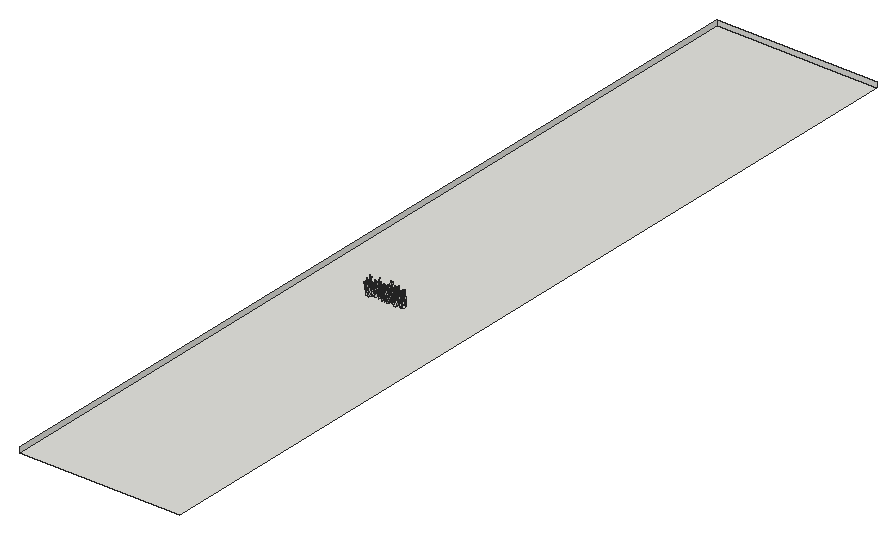
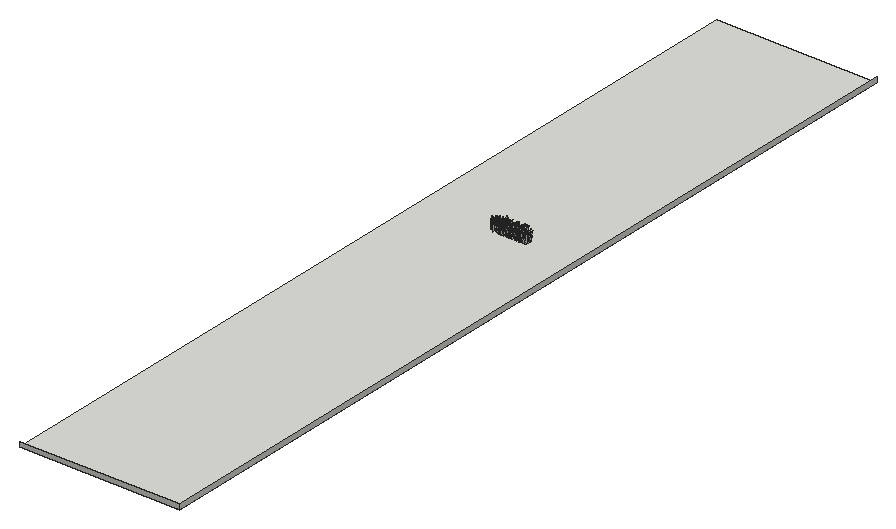
# SketchUp Ruby script. Lengths in inches.
U = 1.inch
M = Sketchup.active_model
def pt(a) = Geom::Point3d.new(a.map { |v| v * U })
def face(e, loops, mat)
  f = e.add_face(loops[0].map { |a| pt(a) })
  loops[1..].each { |l| e.add_face(l.map { |a| pt(a) }).erase! }
  f.material = f.back_material = mat if mat
  f
end
# faces: each face lists its corners as indices into pts; further lists are holes
def faces(e, pts, list, mat = nil) = list.each { |f| face(e, (f[0].is_a?(Array) ? f : [f]).map { |l| l.map { |i| pts[i] } }, mat) }
# xy, xz, yz: faces in a plane at the given z, y or x. An outline is a flat list of corners, or four numbers for a rectangle; further outlines are holes
def ring(l) = l.size == 4 ? [[l[0], l[1]], [l[2], l[1]], [l[2], l[3]], [l[0], l[3]]] : l.each_slice(2).to_a
def flat(e, list, mat, &to3) = list.each { |f| face(e, (f[0].is_a?(Array) ? f : [f]).map { |l| ring(l).map { |u, v| to3.(u, v) } }, mat) }
def xy(e, z, list, mat = nil) = flat(e, list, mat) { |x, y| [x, y, z] }
def xz(e, y, list, mat = nil) = flat(e, list, mat) { |x, z| [x, y, z] }
def yz(e, x, list, mat = nil) = flat(e, list, mat) { |y, z| [x, y, z] }
def lines(e, pts, list) = list.each { |a, b| e.add_line(pt(pts[a]), pt(pts[b])) }
# prism: a flat outline (further loops are holes) pulled along v
def prism(e, loops, v, mat = nil)
  f = face(e, loops, mat); d = Geom::Vector3d.new(v.map { |x| x * U })
  f.pushpull(f.normal.samedirection?(d) ? d.length : -d.length)
end
def box(e, o, s, mat = nil) = prism(e, [[o, [o[0] + s[0], o[1], o[2]], [o[0] + s[0], o[1] + s[1], o[2]], [o[0], o[1] + s[1], o[2]]]], [0, 0, s[2]], mat)
def at(x, y, z, deg = 0) = Geom::Transformation.translation(pt([x, y, z])) * Geom::Transformation.rotation(ORIGIN, Z_AXIS, deg.degrees)
def axes(o, x, y, z) = Geom::Transformation.new([*x, 0, *y, 0, *z, 0, *pt(o).to_a, 1])
def part(name) = M.definitions.add(name)
# library, detail: a bought-in or finely detailed component or shape, given as its bounding box
def library(name, o, s) = part(name).tap { |d| box(d.entities, o, s) }
def detail(e, o, s) = box(e.add_group.entities, o, s)
def put(e, d, t, mat = nil) = e.add_instance(d, t).tap { |i| i.material = mat if mat }
def group(e, t, mat = nil) = e.add_group.tap { |g| g.transformation = t; g.material = mat if mat }.entities
root = M.entities
c1 = part("fur_instance\#9")
p = [[0.8125,0,1.79],[0.67,-0.02,1.48],[0,-0.11,0],[0,0.11,0]]
faces(c1.entities,p,[[0,1,2,3]])
xy(root,-27.625,[[0,5.77,196.6875,1083.4]])
xz(root,1083.4,[[0,-27.625,196.6875,-21.625]])
yz(root,0,[[5.77,-27.625,1083.4,-21.625]])
put(root,c1,axes([103.26,455.89,-27.1],[-3.36255,6.42423,2.20976],[5.77924,4.00105,-2.8377],[3.57129,-0.42595,6.67271]))
put(root,c1,axes([74.56,459.28,-27.1],[-6.62778,2.24684,1.33683],[2.5489,6.36376,1.94128],[0.58185,-2.2841,6.72363]))
put(root,c1,axes([77.29,458.65,-27.1],[2.95876,-6.29379,1.88961],[-6.54545,-2.63888,1.45948],[0.58268,2.31543,6.79971]))
put(root,c1,axes([104.48,458.19,-27.1],[4.99795,-3.82327,1.26682],[-4.01963,-4.86241,1.18375],[-0.25457,1.71502,6.18026]))
put(root,c1,axes([77.6,460.84,-27.1],[6.21031,-0.46369,2.15458],[0.49806,-5.98034,-2.72263],[-2.14689,-2.7287,5.60092]))
put(root,c1,axes([84.37,459.16,-27.1],[-1.75901,-5.06572,0.78099],[-4.97011,1.48393,-1.5689],[-1.25276,1.22556,5.12778]))
put(root,c1,axes([110.68,457.23,-27.1],[-4.80095,-0.85986,1.55653],[-1.24807,4.82151,-1.18603],[1.26668,1.49164,4.73094]))
put(root,c1,axes([102.17,460.42,-27.1],[1.78326,-6.33726,0.7797],[-6.26284,-1.89367,-1.06754],[-1.24322,0.44943,6.49625]))
put(root,c1,axes([85.58,460.71,-27.1],[-2.3415,-4.6423,0.1365],[-4.37976,2.25803,1.66471],[1.54509,-0.63449,4.92568]))
put(root,c1,axes([108.52,457.49,-27.1],[-0.93822,4.8343,1.08723],[4.93478,0.81164,0.64956],[-0.44769,-1.18472,4.88147]))
put(root,c1,axes([69.07,457.7,-27.1],[3.47844,1.93474,0.04271],[1.93521,-3.47755,-0.07868],[0.00093,-0.08952,3.97952]))
put(root,c1,axes([97.93,459.65,-27.1],[4.25123,5.18566,4.75994],[6.35301,-5.22113,0.01405],[-3.03108,-3.67013,6.70551]))
put(root,c1,axes([93.1,457.01,-27.1],[8.11647,0.24258,0.67526],[0.10402,-7.98511,1.61836],[-0.70993,1.60345,7.95719]))
put(root,c1,axes([71.29,455.27,-27.1],[-5.44791,2.04028,1.98238],[0.64646,5.0587,-3.42987],[2.77031,2.83181,4.69878]))
put(root,c1,axes([68.04,456.18,-27.1],[-4.70225,1.57903,0.9136],[0.9953,4.33742,-2.37389],[1.52885,2.03289,4.35536]))
put(root,c1,axes([84.85,458.36,-27.1],[2.54446,5.11145,1.43196],[5.2695,-2.24073,-1.36501],[0.64019,-1.87187,5.54418]))
put(root,c1,axes([110.55,456.91,-27.1],[-4.99347,0.21503,1.45697],[-0.36457,4.80955,-1.95935],[1.42691,1.98134,4.59803]))
put(root,c1,axes([99.07,459.31,-27.1],[-2.91756,2.69263,1.56889],[3.08399,2.80363,0.92331],[0.448,-1.76443,3.86133]))
put(root,c1,axes([73.96,462,-27.1],[5.79186,-5.56058,1.06137],[-5.14067,-5.80215,-2.34538],[-2.37068,-1.00358,7.67886]))
put(root,c1,axes([88.27,459.86,-27.1],[1.0703,-6.74535,2.51722],[-6.58595,-1.94546,-2.41292],[-2.90886,1.9228,6.3893]))
put(root,c1,axes([102.05,460.11,-27.1],[-4.72142,-2.258,0.83052],[-2.14472,4.77905,0.80066],[1.09019,-0.37724,5.17198]))
put(root,c1,axes([68.65,460.14,-27.1],[7.59105,-2.36712,2.02897],[-2.18853,-7.84946,-0.96967],[-2.22043,-0.35586,7.89221]))
put(root,c1,axes([94.5,457.96,-27.1],[4.33311,5.30156,2.10924],[5.44411,-4.63436,0.46433],[-1.70794,-1.32191,6.83131]))
put(root,c1,axes([85.88,459.7,-27.1],[6.5822,-3.48627,0.04021],[-3.46978,-6.5418,0.80411],[0.34104,0.72931,7.40492]))
put(root,c1,axes([72.45,460.19,-27.1],[5.8288,-3.89293,1.62458],[-3.86791,-6.0381,-0.59132],[-1.68328,0.3943,6.98428]))
put(root,c1,axes([71.9,457.04,-27.1],[2.76553,6.92914,2.18566],[6.51494,-3.40021,2.53621],[-3.21647,-0.92942,7.01632]))
put(root,c1,axes([92.13,461.11,-27.1],[7.49694,-1.26912,1.50095],[-0.87324,-7.45265,-1.93987],[-1.76095,-1.70734,7.35199]))
put(root,c1,axes([104.23,458.38,-27.1],[4.8135,2.02359,1.54657],[1.94555,-5.05552,0.55956],[-1.64367,-0.05793,5.19149]))
put(root,c1,axes([98.9,459.67,-27.1],[-0.48959,-3.44443,1.08487],[-3.54488,0.6673,0.51889],[0.68909,0.98557,3.44014]))
put(root,c1,axes([103.34,460.05,-27.1],[-4.54236,-5.48641,0.31776],[-5.31376,4.27953,-2.06985],[-1.40202,1.55551,6.81539]))
put(root,c1,axes([86.07,457.68,-27.1],[3.67219,7.15908,2.03524],[7.27938,-3.92759,0.68132],[-1.55086,-1.48365,8.01705]))
put(root,c1,axes([94.33,458.25,-27.1],[-1.12302,3.48075,0.37457],[3.50037,1.10997,0.18007],[-0.0574,-0.41163,3.65299]))
put(root,c1,axes([67.41,459.81,-27.1],[-3.27496,5.22829,1.96451],[5.47571,2.5569,2.32348],[-1.10043,-2.83671,5.71505]))
put(root,c1,axes([86.4,457.53,-27.1],[4.4489,2.71988,0.66857],[2.4928,-4.41728,1.38241],[-1.27698,0.85286,5.02786]))
put(root,c1,axes([70.7,462.03,-27.1],[0.98136,-7.62341,0.77855],[-7.49654,-1.11781,-1.49599],[-1.58884,0.56543,7.53933]))
put(root,c1,axes([78.21,462.09,-27.1],[0.34985,-8.1007,0.677],[-7.9597,-0.20383,1.67442],[1.6501,0.73429,7.93347]))
put(root,c1,axes([73.08,459.74,-27.1],[-8.06314,0.9505,0.88883],[1.02226,8.07835,0.63476],[0.80526,-0.7379,8.09412]))
put(root,c1,axes([88.92,460.2,-27.1],[-1.01611,-5.1437,1.43202],[-5.3112,0.8243,-0.80778],[-0.54728,1.55038,5.1805]))
put(root,c1,axes([102.97,461.34,-27.1],[2.20766,-6.15742,1.48059],[-5.96151,-2.54967,-1.71445],[-2.13691,0.75174,6.31254]))
put(root,c1,axes([109.11,459.81,-27.1],[3.12486,4.78234,3.10342],[5.39282,-3.6275,0.15986],[-1.8492,-2.49745,5.71052]))
put(root,c1,axes([92.16,458.23,-27.1],[3.27247,4.57721,0.86039],[4.6176,-3.3258,0.13012],[-0.60735,-0.62316,5.62521]))
put(root,c1,axes([87.72,459.5,-27.1],[-7.02647,-2.17808,1.10616],[-2.29777,7.03636,-0.74079],[0.82938,1.04138,7.31892]))
put(root,c1,axes([64.94,460.51,-27.1],[-3.14416,-1.79317,0.28571],[-1.75542,3.14785,0.43854],[0.46429,-0.24163,3.59289]))
put(root,c1,axes([93.54,461.47,-27.1],[-7.87957,1.88276,1.17896],[2.17634,7.41366,2.70618],[0.44527,-2.91806,7.63603]))
put(root,c1,axes([96.59,460.91,-27.1],[-4.94323,1.53486,1.76986],[2.06825,4.80019,1.61379],[1.10026,-2.12747,4.91803]))
put(root,c1,axes([98.81,461.17,-27.1],[-3.02452,-1.82217,1.01563],[-1.34667,3.07159,1.50047],[1.5932,-0.86291,3.19635]))
put(root,c1,axes([96.05,459.14,-27.1],[4.06376,5.39951,0.02576],[4.83357,-3.62337,-3.0294],[2.40665,-1.8401,6.04083]))
put(root,c1,axes([81.59,460.28,-27.1],[4.24659,-4.94069,2.32668],[-5.22174,-4.53655,-0.10277],[-1.59916,1.69313,6.51409]))
put(root,c1,axes([73.99,458.09,-27.1],[-6.21207,0.31771,0.7174],[0.09871,5.99609,-1.80072],[0.77837,1.77522,5.95384]))
put(root,c1,axes([95.84,461.98,-27.1],[4.75134,-2.11282,0.36953],[-1.90852,-4.57438,-1.61505],[-0.97883,-1.33672,4.94275]))
put(root,c1,axes([81.63,458.6,-27.1],[-5.20455,-0.25594,1.25726],[-0.61037,5.11409,-1.48563],[1.12857,1.58561,4.99457]))
put(root,c1,axes([83.66,461.34,-27.1],[-3.27464,-6.78559,1.40651],[-6.92909,3.22889,-0.5548],[0.10135,1.50857,7.51397]))
put(root,c1,axes([74.65,461.13,-27.1],[2.8154,-3.04723,0.70248],[-2.99803,-2.89898,-0.55973],[-0.88933,0.126,4.11081]))
put(root,c1,axes([102.36,459.99,-27.1],[0.25275,3.74041,1.98428],[3.79537,-1.08135,1.55493],[-1.87703,-1.68284,3.41127]))
put(root,c1,axes([101.22,459.71,-27.1],[5.9616,4.7587,3.0284],[5.08757,-6.43918,0.10304],[-2.43578,-1.80245,7.62727]))
put(root,c1,axes([86.71,460.02,-27.1],[-8.26176,0.40654,0.83522],[0.41692,8.30295,0.08258],[0.83009,-0.12394,8.27135]))
put(root,c1,axes([72.48,460.9,-27.1],[6.13982,-1.63324,0.91897],[-1.58888,-6.20592,-0.4139],[-0.99371,-0.16841,6.33984]))
put(root,c1,axes([67.33,460.15,-27.1],[2.36922,2.94645,1.17355],[3.15581,-2.33594,-0.5062],[-0.31572,-1.23846,3.7468]))
put(root,c1,axes([94.24,459.77,-27.1],[-5.6206,-6.05261,0.8091],[-5.56666,4.62654,-4.06048],[-2.5102,3.29256,7.1929]))
put(root,c1,axes([67.6,459.49,-27.1],[2.29816,3.3477,0.63042],[3.39972,-2.30202,-0.16916],[-0.21536,-0.61617,4.05709]))
put(root,c1,axes([72.42,461.59,-27.1],[-0.76172,-5.93829,1.58025],[-5.83151,1.20063,1.7008],[1.93753,1.27903,5.74028]))
put(root,c1,axes([72.01,460.96,-27.1],[0.25447,-5.59234,1.88155],[-5.79418,0.11887,1.13692],[1.11444,1.89496,5.48146]))
put(root,c1,axes([65.3125,459.35,-27.1],[0.45308,4.94253,1.25959],[4.74966,-0.86975,1.70432],[-1.859,-1.01755,4.66145]))
put(root,c1,axes([81.02,460.48,-27.1],[3.81307,5.29138,3.34018],[5.75803,-4.49829,0.55278],[-2.44962,-2.33704,6.49867]))
put(root,c1,axes([111.67,459.09,-27.1],[-1.94953,6.2532,0.70862],[6.08536,1.68405,1.8809],[-1.60411,-1.2111,6.27419]))
put(root,c1,axes([98.69,460.13,-27.1],[1.00735,6.64791,2.58508],[7.07427,-1.26504,0.49655],[-0.91221,-2.46923,6.70544]))
put(root,c1,axes([68.27,462.42,-27.1],[-3.1759,-6.57357,0.78945],[-6.61199,3.10387,-0.75436],[-0.34161,1.03711,7.26148]))
put(root,c1,axes([69.45,459.57,-27.1],[-1.35626,4.67986,0.4324],[4.48876,1.15652,1.56235],[-1.3925,-0.82998,4.61514]))
put(root,c1,axes([88.56,461.75,-27.1],[-3.05463,-4.97038,1.37571],[-5.09206,3.16016,0.11108],[0.81742,1.11209,5.83293]))
put(root,c1,axes([82.23,462.16,-27.1],[-5.80555,-2.80529,1.19859],[-2.69051,5.92298,0.83076],[1.43785,-0.24369,6.39405]))
put(root,c1,axes([96.85,461.16,-27.1],[3.67258,4.04026,0.63824],[3.75616,-2.99162,-2.6759],[1.61937,-2.22383,4.75932]))
put(root,c1,axes([83.24,459.52,-27.1],[2.06268,4.77096,0.10661],[4.57909,-1.94603,-1.50762],[1.34363,-0.69206,4.97431]))
put(root,c1,axes([90,457.62,-27.1],[6.02604,4.35688,0.13616],[4.14402,-5.7981,2.12678],[-1.35204,1.64734,7.12547]))
put(root,c1,axes([103.22,462.74,-27.1],[-5.52274,-3.05851,1.02558],[-2.84433,5.57616,1.31266],[1.52186,-0.67738,6.17511]))
put(root,c1,axes([88.98,459.76,-27.1],[-0.28002,6.79198,1.74012],[7.00527,0.19856,0.35229],[-0.29175,-1.75129,6.78861]))
put(root,c1,axes([72.28,461.87,-27.1],[-3.33376,-1.76985,1.3611],[-1.54667,3.5947,0.88593],[1.61021,-0.21143,3.66899]))
put(root,c1,axes([71.61,459.89,-27.1],[0.20171,6.63601,2.13173],[6.14884,-1.17367,3.07178],[-3.28217,-1.79094,5.8857]))
put(root,c1,axes([99.74,460.84,-27.1],[4.36053,2.62617,0.62372],[2.69593,-4.29581,-0.7602],[-0.13318,-0.97427,5.03319]))
put(root,c1,axes([89.6,460.54,-27.1],[5.1332,2.66859,0.80867],[2.72409,-5.16107,-0.26035],[-0.59552,-0.60587,5.77956]))
put(root,c1,axes([89.5,462.64,-27.1],[2.09335,-3.21544,0.11512],[-3.16402,-2.08217,-0.6229],[-0.58423,-0.24481,3.78592]))
put(root,c1,axes([104.1,462.63,-27.1],[-0.46017,-7.01963,1.64197],[-7.20868,0.46604,-0.02793],[0.07879,1.64032,7.03464]))
put(root,c1,axes([64.98,462.86,-27.1],[-0.80762,-5.18,0.70533],[-5.16495,0.90095,0.70267],[0.80822,0.5814,5.19528]))
put(root,c1,axes([110.33,462.26,-27.1],[-1.30366,-3.70433,0.26528],[-3.50778,1.13584,-1.37745],[-1.21983,0.69265,3.67753]))
put(root,c1,axes([85.72,462.56,-27.1],[-4.15133,-1.53142,0.10873],[-1.49707,4.10736,0.69206],[0.34034,-0.61232,4.37033]))
put(root,c1,axes([74.31,461.63,-27.1],[3.95435,2.54343,1.52337],[2.80761,-4.0284,-0.56212],[-0.95239,-1.31514,4.66797]))
put(root,c1,axes([68.22,465.66,-27.1],[7.18044,-3.7228,0.21814],[-3.29243,-6.55088,-3.42221],[-1.75122,-2.94828,7.32847]))
put(root,c1,axes([86.55,465.32,-27.1],[3.78174,-4.82109,0.17581],[-4.12071,-3.34423,-3.06777],[-2.50869,-1.77444,5.30408]))
put(root,c1,axes([71.15,461.98,-27.1],[5.93404,-1.49093,1.99542],[-1.59561,-6.23409,0.08712],[-1.91274,0.57506,6.11785]))
put(root,c1,axes([110.42,461.14,-27.1],[-0.72601,3.76819,0.7458],[3.80081,0.81458,-0.41575],[0.55615,-0.64789,3.8149]))
put(root,c1,axes([112.07,460.67,-27.1],[-0.60049,6.11637,0.8715],[5.86899,0.29123,2.00004],[-1.92986,-1.0175,5.81123]))
put(root,c1,axes([85.39,464.64,-27.1],[-4.26482,-5.03014,0.77761],[-4.82923,4.31941,1.45497],[1.60794,-0.36894,6.43227]))
put(root,c1,axes([94.93,461.83,-27.1],[4.2362,2.18763,0.04516],[2.18011,-4.21144,-0.49393],[0.18673,-0.4595,4.74206]))
put(root,c1,axes([65.44,461.125,-27.1],[2.30365,5.6713,0.71156],[5.64313,-2.13475,-1.25489],[0.90837,-1.12069,5.9913]))
put(root,c1,axes([83.89,464.3,-27.1],[-3.75985,-4.2409,1.14983],[-3.97997,3.92819,1.47409],[1.86202,-0.16705,5.47255]))
put(root,c1,axes([82.05,463.28,-27.1],[-5.02334,-0.16728,0.55191],[-0.071,4.98153,0.86367],[0.57231,-0.85028,4.95137]))
put(root,c1,axes([93.05,461.35,-27.1],[-5.05417,-1.27819,2.14403],[-1.86511,5.15169,-1.32541],[1.65892,1.89778,5.04199]))
put(root,c1,axes([69.41,462.86,-27.1],[-5.59942,-5.49473,0.70955],[-5.42162,5.22657,-2.3104],[-1.14084,2.13071,7.49717]))
put(root,c1,axes([97.76,463.3,-27.1],[6.10585,-2.9623,2.45846],[-2.96929,-6.55789,-0.52733],[-2.45002,0.56525,6.76598]))
put(root,c1,axes([78,462.82,-27.1],[-6.68615,-0.01766,0.93467],[0.01232,6.74773,0.2156],[0.93476,-0.21523,6.6827]))
put(root,c1,axes([64.89,466.14,-27.1],[-1.50636,-7.45489,0.25307],[-6.77182,1.47502,3.14252],[3.12761,-0.39686,6.92598]))
put(root,c1,axes([84.23,466.12,-27.1],[-5.99255,-5.60768,0.41861],[-5.37957,5.89507,1.95969],[1.63755,-1.155,7.96972]))
put(root,c1,axes([106.72,462.4375,-27.1],[-3.37701,5.49526,1.43426],[5.6473,3.0721,1.52623],[-0.60248,-2.00587,6.26679]))
put(root,c1,axes([85.02,463.15,-27.1],[3.32524,-3.2763,0.88677],[-3.39381,-3.22791,0.80025],[-0.05063,1.1934,4.59902]))
put(root,c1,axes([98.41,462.88,-27.1],[-3.74017,-2.83655,2.38458],[-3.12746,4.23356,0.13062],[1.98777,1.32365,4.69232]))
put(root,c1,axes([76.13,465.88,-27.1],[6.61822,-2.56323,1.80089],[-1.74555,-6.51281,-2.85492],[-2.60123,-2.15113,6.49773]))
put(root,c1,axes([81.86,464.4375,-27.1],[-0.45629,-4.37673,0.42276],[-4.25435,0.54685,1.06962],[1.11127,0.29645,4.26847]))
put(root,c1,axes([98.09,463.51,-27.1],[-0.66847,-3.61729,0.84651],[-3.58891,0.40659,-1.09666],[-0.95975,0.99906,3.51127]))
put(root,c1,axes([72.79,463.15,-27.1],[-3.17,-4.98135,1.74667],[-5.27871,2.99065,-1.05117],[-0.00204,2.03858,5.81015]))
put(root,c1,axes([88.46,463.81,-27.1],[5.05478,-5.09898,2.04992],[-5.28407,-5.27475,-0.09077],[-1.51011,1.38923,7.17929]))
put(root,c1,axes([110.14,463.14,-27.1],[-4.58199,0.67037,2.42399],[0.81188,5.16228,0.10702],[2.38033,-0.47034,4.62953]))
put(root,c1,axes([72.33,464.37,-27.1],[-2.39227,-3.29447,0.41561],[-3.24315,2.42809,0.57931],[0.71291,-0.00928,4.03]))
put(root,c1,axes([92.61,463.44,-27.1],[7.55648,0.00384,2.83421],[0.13477,-8.06186,-0.34839],[-2.831,-0.37353,7.54844]))
put(root,c1,axes([72.91,462.5,-27.1],[4.25693,-2.37845,0.80532],[-2.50825,-3.95225,1.586],[0.11926,1.77474,4.61119]))
put(root,c1,axes([103.84,463.56,-27.1],[-3.08604,-1.58363,1.00431],[-1.62158,3.22493,0.10239],[0.94181,0.36349,3.46714]))
put(root,c1,axes([83.29,464.36,-27.1],[3.25628,-4.96201,1.27437],[-5.08219,-3.31911,0.06246],[-0.64574,1.10043,5.93473]))
put(root,c1,axes([69.7,462.08,-27.1],[-4.60941,2.24833,0.68921],[2.12734,4.63308,-0.88638],[1.00221,0.50623,5.05134]))
put(root,c1,axes([94.92,463.875,-27.1],[-1.35927,-4.19334,1.10265],[-4.18909,0.97193,-1.4678],[-1.11869,1.45561,4.1566]))
put(root,c1,axes([78.83,464.95,-27.1],[7.66511,2.45698,1.17946],[2.70747,-7.26796,-2.45522],[-0.3122,-2.70587,7.66567]))
put(root,c1,axes([77.63,465.21,-27.1],[-4.01189,-2.17426,1.82805],[-1.57492,4.33524,1.69992],[2.36407,-0.80168,4.23473]))
put(root,c1,axes([108.58,462.49,-27.1],[2.96295,7.07925,2.39249],[7.30087,-3.29107,0.69644],[-1.59283,-1.91622,7.64263]))
put(root,c1,axes([71.61,465.22,-27.1],[3.35042,-5.0359,1.55374],[-4.92978,-3.64566,-1.18576],[-1.86322,0.59037,5.93123]))
put(root,c1,axes([107.72,462.6875,-27.1],[-1.2405,4.10694,0.41743],[4.03089,1.11105,1.04764],[-0.89058,-0.69186,4.16031]))
put(root,c1,axes([76.94,464.37,-27.1],[0.54293,-5.17192,1.62827],[-5.42158,-0.49338,0.24063],[0.08095,1.64396,5.19477]))
put(root,c1,axes([70.75,461.55,-27.1],[0.90222,6.95991,0.72818],[6.98982,-0.93156,0.24337],[-0.33621,-0.69025,7.01392]))
put(root,c1,axes([66.5,463.32,-27.1],[-0.43128,5.47544,2.09207],[5.72554,0.84273,-1.02531],[1.25517,-1.9628,5.39585]))
put(root,c1,axes([92.15,463.48,-27.1],[-6.45817,-1.9042,0.82118],[-2.02073,6.38203,-1.093],[0.4658,1.28531,6.64374]))
put(root,c1,axes([100.18,461.98,-27.1],[-5.70534,2.42628,0.74712],[2.22137,5.6608,-1.42016],[1.22905,1.03174,6.03498]))
put(root,c1,axes([64.72,465.14,-27.1],[-3.11694,-3.18155,0.61605],[-3.14817,3.17551,0.47138],[0.76862,0.10457,4.42892]))
put(root,c1,axes([99.35,461.48,-27.1],[2.9038,6.51052,1.10748],[6.2299,-3.10193,1.9005],[-2.1913,-0.1914,6.87074]))
put(root,c1,axes([93.42,461.7,-27.1],[-5.22484,3.83291,1.4033],[3.4058,5.3502,-1.93269],[2.24967,0.80218,6.18505]))
put(root,c1,axes([82.99,466.31,-27.1],[2.63198,-5.20128,0.6124],[-4.94839,-2.69423,-1.6156],[-1.71515,-0.20845,5.60093]))
put(root,c1,axes([98.45,463.17,-27.1],[-2.02202,5.92033,1.45384],[6.05855,1.78151,1.17164],[-0.67672,-1.74024,6.14542]))
put(root,c1,axes([65.25,460.91,-27.1],[-3.2389,7.2108,0.31573],[7.08918,3.2432,-1.34571],[1.35602,0.26802,7.78942]))
put(root,c1,axes([75.41,464.35,-27.1],[-3.7614,2.09395,0.36046],[2.10674,3.58022,1.1859],[-0.27609,-1.20834,4.13841]))
put(root,c1,axes([94.71,465.02,-27.1],[-5.73221,-5.07274,1.73381],[-5.23258,5.8463,-0.19467],[1.1657,1.29813,7.652]))
put(root,c1,axes([98.41,464.04,-27.1],[2.1369,3.02619,1.55246],[3.28055,-2.31782,0.00255],[-0.89775,-1.26656,3.70461]))
put(root,c1,axes([109.38,462.4375,-27.1],[-5.51425,5.90533,1.65371],[5.90522,5.71303,-0.71018],[1.6541,-0.70927,8.04832]))
put(root,c1,axes([65.89,464.3,-27.1],[-2.9488,-2.48385,0.84804],[-2.61567,2.88641,-0.64107],[0.2167,1.04076,3.80183]))
put(root,c1,axes([99.53,461.5625,-27.1],[5.91646,3.40669,0.5347],[3.12979,-5.75065,2.00759],[-1.44773,1.49011,6.52531]))
put(root,c1,axes([85.24,462.12,-27.1],[4.44395,3.96646,1.43413],[3.47391,-4.62357,2.02305],[-2.39195,0.65422,5.60257]))
put(root,c1,axes([67.03,465.44,-27.1],[-3.51503,-1.89548,0.64915],[-1.82323,3.56963,0.55065],[0.83071,-0.18586,3.95538]))
put(root,c1,axes([96.99,461.43,-27.1],[-7.37463,3.18086,0.67882],[2.84062,7.11825,-2.49505],[1.58417,2.04365,7.63399]))
put(root,c1,axes([93.55,462.88,-27.1],[0.65103,4.23875,0.31259],[3.78552,-0.72206,1.9071],[-1.9325,0.01355,3.84107]))
put(root,c1,axes([107.45,463.55,-27.1],[-5.34624,-2.21651,3.3319],[-3.00843,5.89263,-0.90721],[2.6389,2.22728,5.71596]))
put(root,c1,axes([97.42,463,-27.1],[2.23337,6.49328,0.05356],[5.9184,-2.0122,-2.84202],[2.67172,-0.9705,6.25089]))
put(root,c1,axes([102.76,462.95,-27.1],[4.44163,5.80553,0.93246],[5.82565,-4.50337,0.28854],[-0.79717,-0.56325,7.30404]))
put(root,c1,axes([92.73,464.75,-27.1],[4.81991,2.46867,0.79438],[2.57067,-4.76928,-0.77622],[-0.3421,-1.05666,5.35942]))
put(root,c1,axes([69.58,463.08,-27.1],[-0.94911,6.39885,1.08787],[6.32075,1.1611,-1.31509],[1.4754,-0.85797,6.33377]))
put(root,c1,axes([90.01,465.1875,-27.1],[-4.92159,1.07561,1.43405],[1.22896,5.07505,0.41117],[1.30503,-0.72281,5.02095]))
put(root,c1,axes([73.15,465.36,-27.1],[5.8637,3.4963,0.04079],[3.31459,-5.53283,-2.23832],[1.11324,-1.94227,6.44958]))
put(root,c1,axes([77.11,464.31,-27.1],[-5.54363,5.04114,0.10568],[4.92423,5.3789,1.72499],[-1.08457,-1.34553,7.29173]))
put(root,c1,axes([70.92,466.29,-27.1],[6.83601,2.20523,1.02382],[2.40175,-6.59991,-1.82073],[-0.37792,-2.05437,6.94831]))
put(root,c1,axes([66.55,465.47,-27.1],[-2.19445,-3.56039,1.55722],[-3.85398,2.22319,-0.34801],[0.4981,1.5159,4.16783]))
put(root,c1,axes([87.76,464.11,-27.1],[-1.23895,4.11427,0.01816],[3.97981,1.19363,1.09497],[-1.04341,-0.33255,4.15491]))
put(root,c1,axes([87.85,465.29,-27.1],[-5.92651,0.06077,0.05927],[0.05827,5.92175,-0.24529],[0.06173,0.24468,5.92174]))
put(root,c1,axes([84.82,464.91,-27.1],[5.89255,-1.31891,0.46121],[-1.38894,-5.74659,1.31223],[-0.15186,1.38261,5.89404]))
put(root,c1,axes([70.07,464.76,-27.1],[-0.06431,5.36711,1.48252],[5.54585,0.19413,-0.46222],[0.49719,-1.47116,5.34755]))
put(root,c1,axes([76.99,465.38,-27.1],[-4.7956,1.01448,1.55419],[0.95492,5.04106,-0.34401],[1.59148,0.0322,4.88965]))
put(root,c1,axes([91.5625,463.5,-27.1],[4.67368,1.9817,0.84614],[1.46066,-4.3994,2.23565],[-1.58416,1.79011,4.55767]))
put(root,c1,axes([92.39,465.36,-27.1],[-3.14834,2.92622,0.07201],[2.87738,3.07451,0.86494],[-0.53726,-0.68166,4.21031]))
put(root,c1,axes([105.02,466.83,-27.1],[6.65936,-3.07974,1.86174],[-3.09449,-6.89952,-0.34452],[-1.83712,0.458,7.32893]))
put(root,c1,axes([86.79,465.9,-27.1],[-5.29366,2.0126,1.17564],[2.12712,5.36423,0.39489],[0.95291,-0.79376,5.64955]))
put(root,c1,axes([97.7,465.8,-27.1],[-5.4066,3.91291,1.98693],[4.14231,5.59139,0.26032],[1.44915,-1.38406,6.66892]))
put(root,c1,axes([97.77,464.13,-27.1],[-1.13883,5.42731,0.08742],[5.42427,1.13458,0.2244],[-0.2017,-0.13157,5.54096]))
put(root,c1,axes([75.52,465.78,-27.1],[5.25696,-1.00652,0.21452],[-1.02902,-5.15697,1.02054],[-0.01477,1.04274,5.25426]))
put(root,c1,axes([100.52,466.125,-27.1],[-3.60643,-6.53276,3.39182],[-7.2869,3.70246,-0.61691],[1.0404,3.28673,7.43658]))
put(root,c1,axes([92.46,465.48,-27.1],[1.86244,4.7215,0.55373],[4.68693,-1.72429,-1.06173],[0.79484,-0.89561,4.96326]))
put(root,c1,axes([94.17,465.95,-27.1],[-2.76968,5.79414,2.34049],[6.07448,3.09716,-0.47899],[1.46654,-1.88589,6.4042]))
put(root,c1,axes([81.4,466.53,-27.1],[1.95636,4.4496,1.57567],[4.70552,-1.97342,-0.26957],[-0.3738,-1.55425,4.8532]))
put(root,c1,axes([72.83,465.85,-27.1],[-3.84179,0.25674,0.88435],[-0.00822,3.78425,-1.13434],[0.92083,1.10494,3.67947]))
put(root,c1,axes([97.83,466.8,-27.1],[2.36348,3.65871,1.87372],[3.9267,-2.64879,0.21906],[-1.21573,-1.4425,4.3502]))
put(root,c1,axes([86.67,464.93,-27.1],[3.82585,4.29132,1.89582],[3.55577,-4.24822,2.44044],[-3.06039,0.42878,5.20545]))
put(root,c1,axes([74.38,465.21,-27.1],[-4.08665,1.67614,0.95166],[1.15635,3.91687,-1.93308],[1.54207,1.50482,3.97156]))
put(root,c1,axes([74.78,465.25,-27.1],[2.09645,3.63188,0.13416],[3.39461,-2.01213,1.42535],[-1.29816,0.60366,3.94386]))
put(root,c1,axes([73.05,466.04,-27.1],[-4.76791,1.69378,1.39092],[1.4281,4.92716,-1.10462],[1.66255,0.62512,4.93778]))
put(root,c1,axes([65.43,465.83,-27.1],[-5.44191,5.3364,0.6963],[5.36336,5.45938,0.07682],[0.44311,-0.54257,7.6214]))
put(root,c1,axes([93.53,464.43,-27.1],[4.16098,5.56887,0.17793],[5.30628,-4.02846,1.99315],[-1.69922,1.05685,6.65984]))
put(root,c1,axes([75.4375,464.81,-27.1],[-4.827,3.94667,0.05385],[3.76525,4.62978,-1.80751],[1.18405,1.36675,5.96733]))
put(root,c1,axes([97.98,466.61,-27.1],[1.64216,5.46326,1.64146],[5.44457,-2.0108,1.24565],[-1.70244,-1.16093,5.56707]))
put(root,c1,axes([71.1,465.66,-27.1],[0.33819,7.69063,1.05021],[7.70297,-0.20312,-0.99305],[0.95553,-1.08446,7.63374]))
put(root,c1,axes([78.3125,466.77,-27.1],[3.87453,3.49507,1.24049],[3.40824,-4.0629,0.80191],[-1.46226,-0.20898,5.15601]))
put(root,c1,axes([95.03,466.78,-27.1],[-6.05277,2.56522,0.71834],[2.46544,6.06973,-0.90131],[1.00895,0.55714,6.51184]))
put(root,c1,axes([91.22,466.57,-27.1],[-6.67208,0.88571,0.68005],[0.61302,6.34873,-2.25421],[0.93335,2.16166,6.3419]))
put(root,c1,axes([88.92,466.6,-27.1],[4.06044,6.49572,1.60929],[6.19974,-4.35997,1.95581],[-2.5194,-0.26008,7.4065]))
put(root,c1,axes([85.96,466.32,-27.1],[7.23662,0.86237,3.59764],[-0.54989,-7.56504,2.91946],[-3.65846,2.84288,6.67751]))
